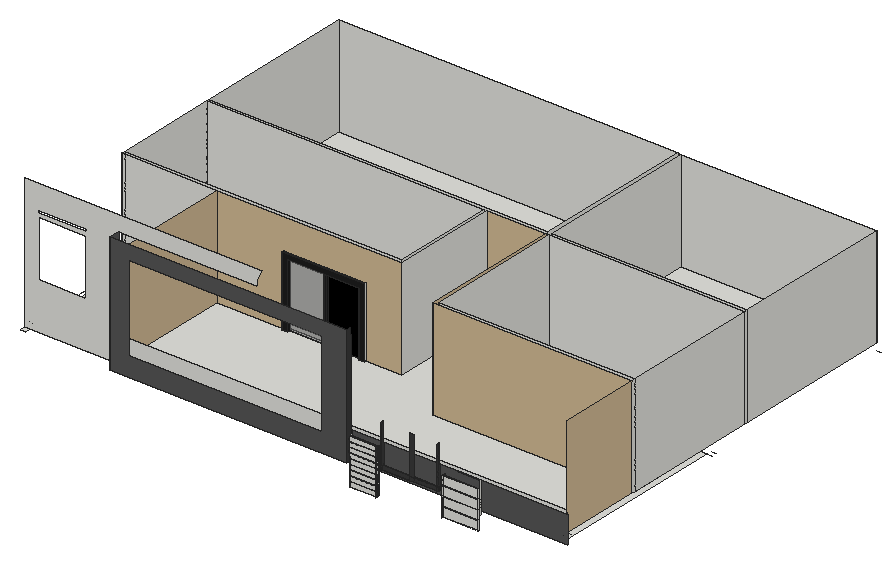
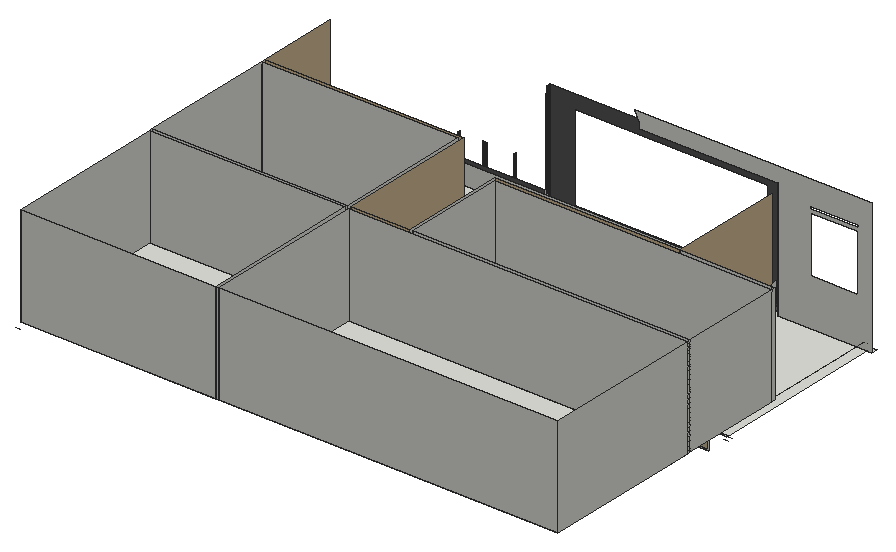
# SketchUp Ruby script. Lengths in inches.
U = 1.inch
M = Sketchup.active_model
def pt(a) = Geom::Point3d.new(a.map { |v| v * U })
def face(e, loops, mat)
  f = e.add_face(loops[0].map { |a| pt(a) })
  loops[1..].each { |l| e.add_face(l.map { |a| pt(a) }).erase! }
  f.material = f.back_material = mat if mat
  f
end
# faces: each face lists its corners as indices into pts; further lists are holes
def faces(e, pts, list, mat = nil) = list.each { |f| face(e, (f[0].is_a?(Array) ? f : [f]).map { |l| l.map { |i| pts[i] } }, mat) }
# xy, xz, yz: faces in a plane at the given z, y or x. An outline is a flat list of corners, or four numbers for a rectangle; further outlines are holes
def ring(l) = l.size == 4 ? [[l[0], l[1]], [l[2], l[1]], [l[2], l[3]], [l[0], l[3]]] : l.each_slice(2).to_a
def flat(e, list, mat, &to3) = list.each { |f| face(e, (f[0].is_a?(Array) ? f : [f]).map { |l| ring(l).map { |u, v| to3.(u, v) } }, mat) }
def xy(e, z, list, mat = nil) = flat(e, list, mat) { |x, y| [x, y, z] }
def xz(e, y, list, mat = nil) = flat(e, list, mat) { |x, z| [x, y, z] }
def yz(e, x, list, mat = nil) = flat(e, list, mat) { |y, z| [x, y, z] }
def lines(e, pts, list) = list.each { |a, b| e.add_line(pt(pts[a]), pt(pts[b])) }
# prism: a flat outline (further loops are holes) pulled along v
def prism(e, loops, v, mat = nil)
  f = face(e, loops, mat); d = Geom::Vector3d.new(v.map { |x| x * U })
  f.pushpull(f.normal.samedirection?(d) ? d.length : -d.length)
end
def box(e, o, s, mat = nil) = prism(e, [[o, [o[0] + s[0], o[1], o[2]], [o[0] + s[0], o[1] + s[1], o[2]], [o[0], o[1] + s[1], o[2]]]], [0, 0, s[2]], mat)
def at(x, y, z, deg = 0) = Geom::Transformation.translation(pt([x, y, z])) * Geom::Transformation.rotation(ORIGIN, Z_AXIS, deg.degrees)
def axes(o, x, y, z) = Geom::Transformation.new([*x, 0, *y, 0, *z, 0, *pt(o).to_a, 1])
def part(name) = M.definitions.add(name)
# library, detail: a bought-in or finely detailed component or shape, given as its bounding box
def library(name, o, s) = part(name).tap { |d| box(d.entities, o, s) }
def detail(e, o, s) = box(e.add_group.entities, o, s)
def put(e, d, t, mat = nil) = e.add_instance(d, t).tap { |i| i.material = mat if mat }
def group(e, t, mat = nil) = e.add_group.tap { |g| g.transformation = t; g.material = mat if mat }.entities
root = M.entities
M.materials.add("[0137_Black]").color = [0, 0, 0]
M.materials.add("[Color M06]").color = [86, 86, 86]
M.materials.add("[Color M07]").color = [58, 58, 58]
M.materials.add("[Color M08]").color = [30, 30, 30]
M.materials.add("[Formica Beige]").color = [211, 187, 149]
M.materials.add("[Quartz Light Brown]").color = [199, 184, 152]
M.materials.add("[Translucent Glass Gray]").color = [128, 128, 128]
M.materials["[Translucent Glass Gray]"].alpha = 0.5
M.materials.add("[Wood Veneer 01]").color = [120, 70, 37]
xy(root,139.68,[[595.0625,21.0625,644.47,22.14]])
xy(root,143.6,[[419.8,347.125,426.4375,350.125]])
xy(root,143.6,[[352.52,347.125,419.8,350.125],[426.4375,347.125,487.09,350.125]],"[Color M08]")
xy(root,151.99,[[514.29,350.125,608.23,353.125]],"[Wood Veneer 01]")
xy(root,152.83,[[343.29,347.125,496.31,350.125]],"[Color M08]")
xy(root,175.47,[[595.0625,20.83,644.47,22.09]])
xy(root,176.43,[[595.0625,20.82,644.47,22.14]])
xy(root,180,[[0,27,9,36],[169.75,27,169.75,36,9,36,9,347.125,25.58,347.125,25.58,346.125,99.55,346.125,99.55,345.8125,220.94,345.8125,220.94,350.125,972.875,350.125,972.875,27],[99.55,345.8125,167.26,350.125],[167.26,345.8125,220.94,350.125],[25.58,346.125,99.55,350.125],
  [9,347.125,25.58,350.125],[25.58,350.125,99.55,359.125],[25.58,359.125,99.55,398.125]])
xy(root,180,[[169.75,15,595.0625,27]],"[Color M06]")
xy(root,192,[[180.5,36,973.625,36,973.625,180.6875,617,180.6875,617,330.04,614,330.04,614,366.04,617,366.04,617,433.1875,575.92,433.1875,575.92,430.1875,539.92,430.1875,539.92,433.1875,512,433.1875,512,242.9375,446.86,242.9375,446.86,239.9375,436.37,239.9375,436.37,242.9375,378.48,242.9375,378.48,239.9375,373.18,239.9375,373.18,242.9375,309.99,242.9375,309.99,239.9375,299.5,239.9375,299.5,242.9375,180.5,242.9375],[617,180.6875,617,330.04,614,330.04,614,366.04,617,366.04,617,433.1875,512,433.1875,512,242.9375,9,242.9375,9,248.9375,506,248.9375,506,433.1875,9,433.1875,9,439.29,617,439.29,617,729,623,729,623,439.1875,973.625,439.1875,973.625,433.1875,623,433.1875,623,186.6875,973.625,186.6875,973.625,180.6875],[623,186.6875,973.625,433.1875],[299.5,239.9375,309.99,242.9375],[373.18,239.9375,378.48,242.9375],
  [436.37,239.9375,446.86,242.9375],[9,248.9375,506,433.1875],[539.92,430.1875,575.92,433.1875],[623,439.1875,973.625,729],[9,439.29,617,729]])
xz(root,15,[[[169.75,180,595.0625,393.5625],[204.375,214.25,549.5625,368.875]]],"[Color M06]")
xz(root,27,[[595.0625,180,982.625,180,982.625,228,825.84,228,825.84,227.94,595.0625,227.94]],"[Color M06]")
xz(root,36,[[[0,180,169.75,180,169.75,393.5625,416.9375,393.5625,416.9375,402.25,426.66,420,0,420],[25.4,264.24,110.21,366.11],[24.53,371.68,111.9,376.93]],[180.5,192,973.625,228]])
xz(root,180.6875,[[617,192,973.625,372]],"[Formica Beige]")
xz(root,186.6875,[[623,192,973.625,372]])
xz(root,239.9375,[[299.5,192,309.99,192,309.99,306.75,436.37,306.75,436.37,192,446.86,192,446.86,317.24,299.5,317.24],[373.18,192,378.48,306.75]],"[Color M08]")
xz(root,242.9375,[[9,192,14.75,372],[14.75,192,180.5,372]])
xz(root,242.9375,[[378.48,192,436.37,306.75]],"[0137_Black]")
xz(root,242.9375,[[180.5,192,299.5,192,299.5,317.24,446.86,317.24,446.86,192,512,192,512,372,180.5,372]],"[Formica Beige]")
xz(root,242.9375,[[309.99,192,373.18,306.75]],"[Translucent Glass Gray]")
xz(root,248.9375,[[9,192,506,372]])
xz(root,330.04,[[614,192,617,276]],"[Wood Veneer 01]")
xz(root,346.125,[[[44.38,142.05,78.26,168.55],[46.57,144.24,76.07,166.36]]])
xz(root,346.125,[[46.57,144.24,76.07,166.36]],"[Quartz Light Brown]")
xz(root,366.04,[[614,192,617,276]],"[Wood Veneer 01]")
xz(root,430.1875,[[[539.92,192,575.92,276],[548.71,236.42,547.11,236.63,545.62,237.25,544.34,238.24,543.36,239.52,542.74,241.01,542.53,242.61,542.74,244.21,543.36,245.7,544.34,246.99,545.62,247.97,547.11,248.59,548.71,248.8,550.32,248.59,551.81,247.97,553.09,246.99,554.07,245.7,554.69,244.21,554.9,242.61,554.69,241.01,554.07,239.52,553.09,238.24,551.81,237.25,550.32,236.63]]],"[Wood Veneer 01]")
xz(root,433.1875,[[9,192,506,372],[539.92,192,575.92,276],[623,192,973.625,372]])
xz(root,433.1875,[[512,192,539.92,192,539.92,276,575.92,276,575.92,192,617,192,617,372,512,372]],"[Formica Beige]")
xz(root,439.1875,[[623,192,973.625,372]])
xz(root,439.29,[[9,192,617,372]])
xz(root,729,[[9,192,617,372],[617,192,623,372],[623,192,973.625,372]])
yz(root,9,[[242.9375,192,248.9375,372],[248.9375,192,433.1875,372],[433.1875,192,439.29,372],[439.29,192,729,372]])
yz(root,169.75,[[15,180,36,393.5625]],"[Color M06]")
yz(root,180.5,[[27,192,36,228]])
yz(root,180.5,[[36,192,242.9375,372]],"[Formica Beige]")
yz(root,299.5,[[239.9375,192,242.9375,317.24]],"[Color M08]")
yz(root,309.99,[[239.9375,192,242.9375,306.75]],"[Color M08]")
yz(root,373.18,[[239.9375,192,242.9375,306.75]],"[Color M08]")
yz(root,378.48,[[239.9375,192,242.9375,306.75]],"[Color M08]")
yz(root,436.37,[[239.9375,192,242.9375,306.75]],"[Color M08]")
yz(root,446.86,[[239.9375,192,242.9375,317.24]])
yz(root,506,[[248.9375,192,433.1875,372]])
yz(root,512,[[242.9375,192,433.1875,372]])
yz(root,539.92,[[430.1875,192,433.1875,276]],"[Wood Veneer 01]")
yz(root,575.92,[[430.1875,192,433.1875,276]])
yz(root,595.0625,[[21.0625,139.68,21.01,147.9,22.09,147.91,22.14,139.68],[21,148.86,20.95,157.09,22.09,157.1,22.14,148.87],[20.94,158.05,20.89,166.28,22.09,166.29,22.14,158.06],[20.88,167.24,20.83,175.47,22.09,175.47,22.14,167.25],[20.82,176.43,20.8,179.99,22.12,180,22.14,176.43],
  [20.8,179.99,20.8,180,20.77,184.65,22.09,184.66,22.12,180],[24.3125,180,27,180,27,228,24,227.98],[20.76,185.61,20.71,193.84,22.09,193.85,22.14,185.62],[20.7,194.8,20.65,203.03,22.09,203.04,22.14,194.81],[20.65,203.99,20.59,212.21,22.09,212.22,22.14,204],
  [20.59,213.17,20.53,221.4,22.09,221.41,22.14,213.18]])
yz(root,595.0625,[[15,180,24.3125,180,23.0625,371.92,22.92,393.5625,15,393.5625]],"[Color M07]")
yz(root,614,[[[330.04,192,366.04,276],[355.38,232.08,361.82,235.8,361.82,243.23,355.38,246.95,348.94,243.23,348.94,235.8]]],"[Wood Veneer 01]")
yz(root,617,[[439.29,192,729,372]])
yz(root,617,[[180.6875,192,180.6875,372,433.1875,372,433.1875,192,366.04,192,366.04,276,330.04,276,330.04,192]],"[Formica Beige]")
yz(root,623,[[186.6875,192,433.1875,372],[439.1875,192,729,372]])
yz(root,644.47,[[21.0625,139.68,21.01,147.9,21.52,147.91,21.57,139.68],[21.57,139.68,21.52,147.91,22.09,147.91,22.14,139.68],[22.14,139.68,22.09,147.91,24.52,147.93,24.57,139.7],[21.52,147.91,21.52,148.87,22.14,148.87,24.52,148.89,24.52,147.93,22.09,147.91],[21,148.86,20.95,157.09,21.46,157.1,21.52,148.87],
  [21.52,148.87,21.46,157.1,22.09,157.1,22.14,148.87],[22.14,148.87,22.09,157.1,24.46,157.11,24.52,148.89],[21.46,157.1,21.46,158.05,22.14,158.06,24.46,158.07,24.46,157.11,22.09,157.1],[20.94,158.05,20.89,166.28,21.4,166.28,21.46,158.05],[21.46,158.05,21.4,166.28,22.09,166.29,22.14,158.06],
  [22.14,158.06,22.09,166.29,24.4,166.3,24.46,158.07],[21.4,166.28,21.4,167.24,22.14,167.25,24.4,167.26,24.4,166.3,22.09,166.29],[20.88,167.24,20.83,175.47,21.34,175.47,21.4,167.24],[21.4,167.24,21.34,175.47,22.09,175.47,22.14,167.25],[22.14,167.25,22.09,175.47,24.34,175.49,24.4,167.26],
  [21.34,175.47,21.34,176.43,22.14,176.43,24.34,176.45,24.34,175.49,22.09,175.47],[20.82,176.43,20.77,184.65,21.28,184.66,21.34,176.43],[21.34,176.43,21.28,184.66,22.09,184.66,22.14,176.43],[22.14,176.43,22.09,184.66,24.28,184.68,24.34,176.45],[21.28,184.66,21.28,185.62,22.14,185.62,24.28,185.64,24.28,184.68,22.09,184.66],
  [20.76,185.61,20.71,193.84,21.22,193.84,21.28,185.62],[21.28,185.62,21.22,193.84,22.09,193.85,22.14,185.62],[22.14,185.62,22.09,193.85,24.22,193.86,24.28,185.64],[21.22,193.84,21.22,194.8,22.14,194.81,24.22,194.82,24.22,193.86,22.09,193.85],[20.7,194.8,20.65,203.03,21.16,203.03,21.22,194.8],
  [21.22,194.8,21.16,203.03,22.09,203.04,22.14,194.81],[22.14,194.81,22.09,203.04,24.16,203.05,24.22,194.82],[21.16,203.03,21.16,203.99,22.14,204,24.16,204.01,24.16,203.05,22.09,203.04],[20.65,203.99,20.59,212.21,21.1,212.22,21.16,203.99],[21.16,203.99,21.1,212.22,22.09,212.22,22.14,204],
  [22.14,204,22.09,212.22,24.1,212.24,24.16,204.01],[21.1,212.22,21.1,213.18,22.14,213.18,24.1,213.2,24.1,212.24,22.09,212.22],[20.59,213.17,20.53,221.4,21.04,221.4,21.1,213.18],[21.1,213.18,21.04,221.4,22.09,221.41,22.14,213.18],[22.14,213.18,22.09,221.41,24.04,221.42,24.1,213.2]])
yz(root,644.47,[[18.57,139.66,18.52,147.89,21.01,147.9,21.0625,139.68],[18.52,147.89,18.52,148.85,21,148.86,21.52,148.87,21.52,147.91,21.01,147.9],[18.52,148.85,18.46,157.08,20.95,157.09,21,148.86],[18.46,157.08,18.46,158.03,20.94,158.05,21.46,158.05,21.46,157.1,20.95,157.09],[18.46,158.03,18.4,166.26,20.89,166.28,20.94,158.05],
  [18.4,166.26,18.4,167.22,20.88,167.24,21.4,167.24,21.4,166.28,20.89,166.28],[18.4,167.22,18.34,175.45,20.83,175.47,20.88,167.24],[18.34,175.45,18.34,176.41,20.82,176.43,21.34,176.43,21.34,175.47,20.83,175.47],[18.34,176.41,18.28,184.64,20.77,184.65,20.82,176.43],[18.28,184.64,18.28,185.6,20.76,185.61,21.28,185.62,21.28,184.66,20.77,184.65],
  [18.28,185.6,18.22,193.82,20.71,193.84,20.76,185.61],[18.22,193.82,18.22,194.78,20.7,194.8,21.22,194.8,21.22,193.84,20.71,193.84],[18.22,194.78,18.16,203.01,20.65,203.03,20.7,194.8],[18.16,203.01,18.16,203.97,20.65,203.99,21.16,203.99,21.16,203.03,20.65,203.03],[18.16,203.97,18.1,212.2,20.59,212.21,20.65,203.99],
  [18.1,212.2,18.1,213.16,20.59,213.17,21.1,213.18,21.1,212.22,20.59,212.21],[18.1,213.16,18.04,221.39,20.53,221.4,20.59,213.17]],"[Color M07]")
yz(root,653.47,[[21.26,187.5,22.78,187.51,22.73,194.62,21.22,194.61]])
yz(root,653.47,[[18.26,187.48,21.26,187.5,21.22,194.61,18.22,194.59],[22.78,187.51,24.26,187.52,24.22,194.63,22.73,194.62],[18.22,194.59,21.22,194.61,20.77,263.62,17.77,263.6],[21.22,194.61,22.73,194.62,24.22,194.63,23.77,263.64,22.78,263.63,20.77,263.62]],"[Color M07]")
yz(root,753.91,[[21.26,187.5,21.22,194.61,22.73,194.62,22.78,187.51],[22.78,187.51,22.73,194.62,24.22,194.63,24.26,187.52]])
yz(root,753.91,[[18.26,187.48,18.22,194.59,21.22,194.61,21.26,187.5],[18.22,194.59,17.77,263.6,20.77,263.62,21.22,194.61],[21.22,194.61,20.77,263.62,22.78,263.63,23.77,263.64,24.22,194.63,22.73,194.62]],"[Color M07]")
yz(root,762.91,[[18.51,149.58,19.95,149.59,21.51,149.6,21.5,150.74,19.94,150.73,18.5,150.72],[21.51,149.6,22.09,149.6,24.51,149.61,24.5,150.76,22.1875,150.75,21.5,150.74],[18.5,150.72,19.94,150.73,19.84,166.33,18.4,166.33],[19.94,150.73,21.5,150.74,21.4,166.34,19.84,166.33],[21.5,150.74,22.1875,150.75,22.09,166.35,21.4,166.34],
  [22.1875,150.75,24.5,150.76,24.4,166.36,22.09,166.35],[18.4,166.33,19.84,166.33,21.4,166.34,21.39,167.49,19.83,167.48,18.39,167.47],[21.4,166.34,22.09,166.35,24.4,166.36,24.39,167.51,22.1875,167.5,21.39,167.49],[18.39,167.47,19.83,167.48,19.73,183.08,18.29,183.07],[19.83,167.48,21.39,167.49,21.29,183.09,19.73,183.08],
  [21.39,167.49,22.1875,167.5,22.09,183.1,21.29,183.09],[22.1875,167.5,24.39,167.51,24.29,183.11,22.09,183.1],[18.29,183.07,19.73,183.08,21.29,183.09,21.28,184.43,19.72,184.42,18.28,184.41],[21.29,183.09,22.09,183.1,24.29,183.11,24.28,184.45,22.1875,184.44,21.28,184.43],[18.28,184.41,19.72,184.42,19.62,200.02,18.18,200.01],
  [19.72,184.42,21.28,184.43,21.18,200.03,19.62,200.02],[21.28,184.43,22.1875,184.44,22.09,200.04,21.18,200.03],[22.1875,184.44,24.28,184.45,24.18,200.05,22.09,200.04],[24.28,184.45,24.18,200.05,24.27,200.05,24.375,184.45],[18.18,200.01,19.62,200.02,21.18,200.03,21.17,201.37,19.61,201.36,18.17,201.35],
  [21.18,200.03,21.17,201.37,22.1875,201.37,24.17,201.39,24.18,200.05,22.09,200.04],[18.17,201.35,19.61,201.36,19.51,216.96,18.07,216.95],[19.61,201.36,21.17,201.37,21.07,216.97,19.51,216.96],[21.17,201.37,22.1875,201.37,22.09,216.97,21.07,216.97],[22.1875,201.37,22.09,216.97,24.07,216.99,24.17,201.39]])
yz(root,825.84,[[19.94,150.73,22.1875,150.75,22.09,166.35,19.84,166.33],[19.83,167.48,22.1875,167.5,22.09,183.1,19.73,183.08],[24.36,172.42,27.36,172.4375,27,227.94,27,228,24,227.98,24.18,200.05,24.28,184.45],[19.72,184.42,22.1875,184.44,22.09,200.04,19.62,200.02],[22.1875,184.44,24.28,184.45,24.18,200.05,22.09,200.04],
  [24.28,184.45,24.375,184.45,24.27,200.05,24.18,200.05],[19.61,201.36,22.1875,201.37,22.09,216.97,19.51,216.96]])
yz(root,973.625,[[35.0625,192,36,228],[180.6875,192,186.6875,372],[186.6875,192,433.1875,372],[433.1875,192,439.1875,372],[439.1875,192,729,372]])
yz(root,973.625,[[36,192,36,228,35.0625,228,35.0625,372,180.6875,372,180.6875,192]],"[Formica Beige]")
p = [[595.0625,21.01,147.9],[595.0625,21.0625,139.68],[644.47,21.0625,139.68],[644.47,21.01,147.9],[595.0625,22.14,139.68],[595.0625,22.09,147.91],
  [644.47,22.09,147.91],[644.47,22.14,139.68],[644.47,21.52,147.91],[595.0625,20.95,157.09],[595.0625,21,148.86],[644.47,21,148.86],
  [644.47,20.95,157.09],[595.0625,22.14,148.87],[644.47,22.14,148.87],[644.47,21.52,148.87],[595.0625,22.09,157.1],[644.47,22.09,157.1],
  [825.84,22.09,149.6],[762.91,22.09,149.6],[762.91,21.51,149.6],[762.91,19.95,149.59],[825.84,19.95,149.59],[762.91,19.84,166.33],
  [762.91,19.94,150.73],[825.84,19.94,150.73],[825.84,19.84,166.33],[762.91,22.1875,150.75],[825.84,22.1875,150.75],[762.91,21.5,150.74],
  [762.91,22.09,166.35],[825.84,22.09,166.35],[644.47,21.46,157.1],[595.0625,20.89,166.28],[595.0625,20.94,158.05],[644.47,20.94,158.05],
  [644.47,20.89,166.28],[595.0625,22.14,158.06],[644.47,22.14,158.06],[644.47,21.46,158.05],[595.0625,22.09,166.29],[644.47,22.09,166.29],
  [762.91,21.4,166.34],[644.47,21.4,166.28],[595.0625,20.83,175.47],[595.0625,20.88,167.24],[644.47,20.88,167.24],[644.47,20.83,175.47],
  [595.0625,22.14,167.25],[644.47,22.14,167.25],[644.47,21.4,167.24],[595.0625,22.09,175.47],[644.47,22.09,175.47],[762.91,19.73,183.08],
  [762.91,19.83,167.48],[825.84,19.83,167.48],[825.84,19.73,183.08],[762.91,22.1875,167.5],[825.84,22.1875,167.5],[762.91,21.39,167.49],
  [762.91,22.09,183.1],[825.84,22.09,183.1],[784.34,27.36,172.4375],[784.34,27,227.94],[825.84,27,227.94],[825.84,27.36,172.4375],
  [595.0625,20.8,179.99],[595.0625,20.82,176.43],[644.47,20.82,176.43],[644.47,20.77,184.65],[595.0625,20.77,184.65],[595.0625,20.8,180],
  [595.0625,22.14,176.43],[595.0625,22.12,180],[595.0625,22.09,184.66],[644.47,22.09,184.66],[644.47,22.14,176.43],[762.91,21.29,183.09],
  [762.91,19.62,200.02],[762.91,19.72,184.42],[825.84,19.72,184.42],[825.84,19.62,200.02],[762.91,22.1875,184.44],[825.84,22.1875,184.44],
  [762.91,21.28,184.43],[762.91,22.09,200.04],[825.84,22.09,200.04],[762.91,24.28,184.45],[762.91,24.375,184.45],[825.84,24.375,184.45],
  [825.84,24.28,184.45],[762.91,24.27,200.05],[825.84,24.27,200.05],[644.47,21.28,184.66],[595.0625,20.71,193.84],[595.0625,20.76,185.61],
  [644.47,20.76,185.61],[644.47,20.71,193.84],[595.0625,22.14,185.62],[644.47,22.14,185.62],[644.47,21.28,185.62],[595.0625,22.09,193.85],
  [644.47,22.09,193.85],[653.47,21.26,187.5],[703.69,21.26,187.5],[703.69,21.22,194.61],[653.47,21.22,194.61],[710.84,21.26,187.5],
  [710.84,21.22,194.61],[753.91,21.22,194.61],[753.91,21.26,187.5],[653.47,22.78,187.51],[703.69,22.78,187.51],[710.84,22.78,187.51],
  [753.91,22.78,187.51],[653.47,22.73,194.62],[703.69,22.73,194.62],[710.84,22.73,194.62],[753.91,22.73,194.62],[644.47,21.22,193.84],
  [703.69,20.77,263.62],[710.84,20.77,263.62],[595.0625,20.65,203.03],[595.0625,20.7,194.8],[644.47,20.7,194.8],[644.47,20.65,203.03],
  [595.0625,22.14,194.81],[644.47,22.14,194.81],[644.47,21.22,194.8],[595.0625,22.09,203.04],[644.47,22.09,203.04],[762.91,21.18,200.03],
  [825.84,24.18,200.05],[762.91,24.18,200.05],[762.91,19.51,216.96],[762.91,19.61,201.36],[825.84,19.61,201.36],[825.84,19.51,216.96],
  [762.91,22.1875,201.37],[825.84,22.1875,201.37],[762.91,21.17,201.37],[762.91,22.09,216.97],[825.84,22.09,216.97],[644.47,21.16,203.03],
  [595.0625,20.59,212.21],[595.0625,20.65,203.99],[644.47,20.65,203.99],[644.47,20.59,212.21],[595.0625,22.14,204],[644.47,22.14,204],
  [644.47,21.16,203.99],[595.0625,22.09,212.22],[644.47,22.09,212.22],[644.47,21.1,212.22],[595.0625,20.53,221.4],[595.0625,20.59,213.17],
  [644.47,20.59,213.17],[644.47,20.53,221.4],[595.0625,22.14,213.18],[644.47,22.14,213.18],[644.47,21.1,213.18],[595.0625,22.09,221.41],
  [644.47,22.09,221.41],[972.875,359.125,180],[982.625,359.125,180],[9,359.125,180],[0,359.125,180],[9,350.125,180],
  [0,350.125,180],[972.875,729,180],[982.625,729,180],[972.875,350.125,180],[982.625,350.125,180],[14.75,242.9375,192],
  [14.75,36,192],[9,36,192],[9,36.875,192],[180.5,27,192],[595.0625,27,192],[169.75,27,192],
  [973.625,35.0625,192],[973.625,27,192],[982.625,35.0625,192],[446.86,242.9375,181.51],[446.86,242.9375,192],[299.5,242.9375,192],
  [299.5,242.9375,181.51]]
faces(root,p,[[0,1,2,3],[4,5,6,7],[6,5,0,3,8],[9,10,11,12],[13,14,15,11,10],[13,16,17,14],[18,19,20,21,22],[23,24,25,26],
  [27,28,25,24,29],[27,30,31,28],[17,16,9,12,32],[33,34,35,36],[37,38,39,35,34],[37,40,41,38],[31,30,42,23,26],[41,40,33,36,43],
  [44,45,46,47],[48,49,50,46,45],[48,51,52,49],[53,54,55,56],[57,58,55,54,59],[57,60,61,58],[62,63,64,65],[66,67,68,69,70,71],
  [72,73,74,75,76],[61,60,77,53,56],[78,79,80,81],[82,83,80,79,84],[82,85,86,83],[83,82,87,88,89,90],[88,91,92,89],[75,74,70,69,93],
  [94,95,96,97],[98,99,100,96,95],[98,101,102,99],[112,113,107,104],[112,111,115,116,117,118,114,113],[102,101,94,97,119],[117,116,105,108],[122,123,124,125],
  [126,127,128,124,123],[126,129,130,127],[86,85,131,78,81],[85,86,132,92,91,133],[134,135,136,137],[138,139,136,135,140],[138,141,142,139],[130,129,122,125,143],
  [144,145,146,147],[148,149,150,146,145],[148,151,152,149],[152,151,144,147,153],[154,155,156,157],[158,159,160,156,155],[158,161,162,159]])
faces(root,p,[[103,104,105,106],[107,108,105,104],[109,108,107,110],[111,112,104,103],[113,114,110,107],[120,105,108,121],[116,115,106,105],[118,117,108,109]],"[Color M07]")
lines(root,p,[[163,164],[165,166],[167,168],[169,170],[171,172],[173,174],[175,176],[177,178],[177,179],[180,181],[180,182],[183,184],
  [185,186]])
